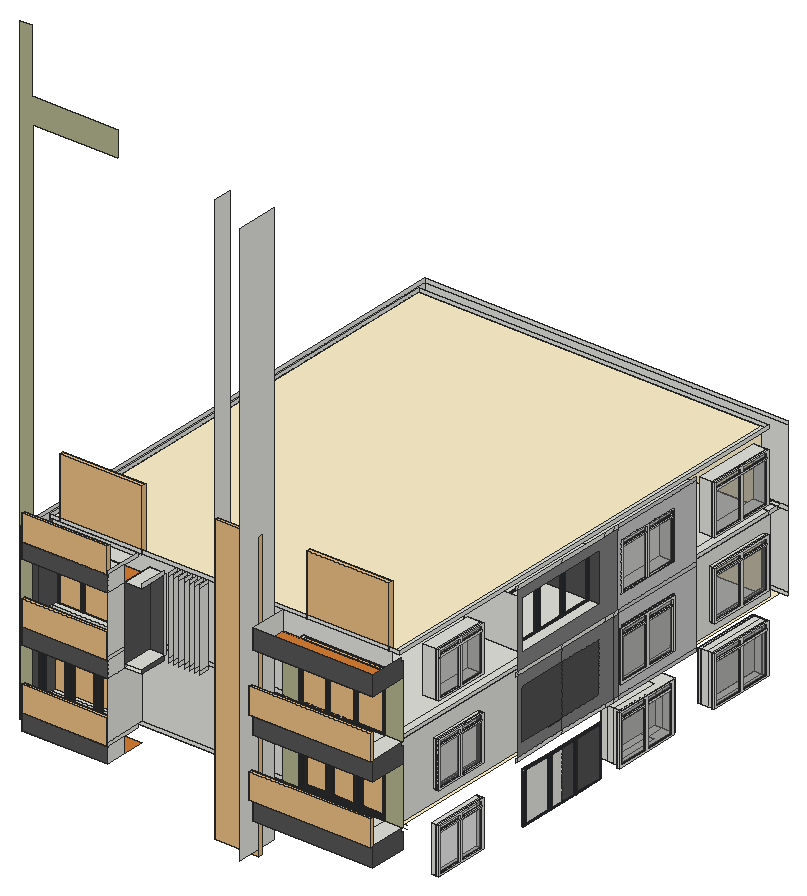
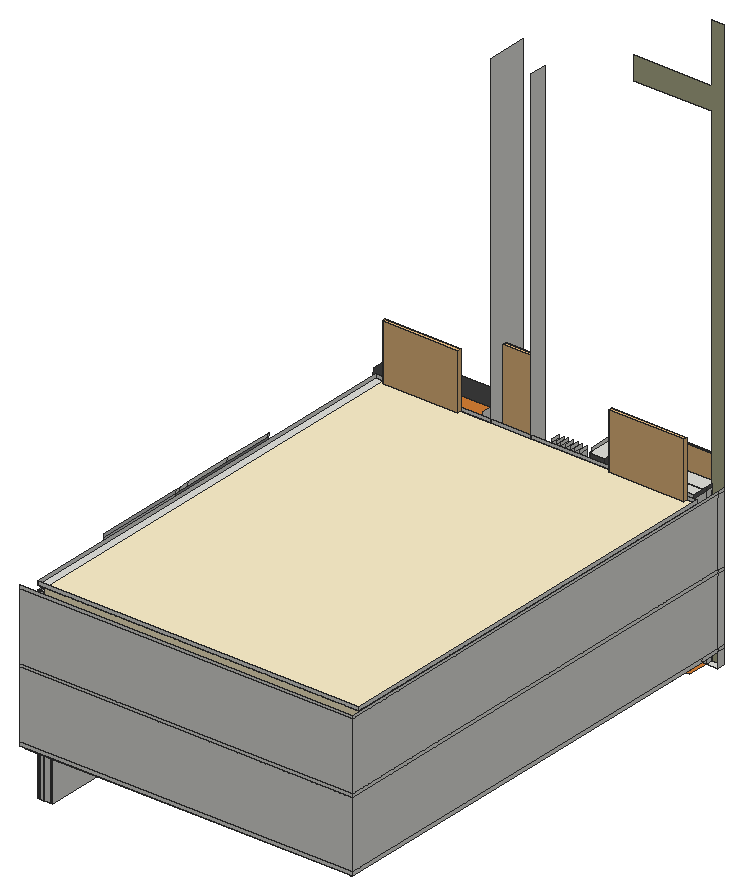
# SketchUp Ruby script. Lengths in inches.
U = 1.inch
M = Sketchup.active_model
def pt(a) = Geom::Point3d.new(a.map { |v| v * U })
def face(e, loops, mat)
  f = e.add_face(loops[0].map { |a| pt(a) })
  loops[1..].each { |l| e.add_face(l.map { |a| pt(a) }).erase! }
  f.material = f.back_material = mat if mat
  f
end
# faces: each face lists its corners as indices into pts; further lists are holes
def faces(e, pts, list, mat = nil) = list.each { |f| face(e, (f[0].is_a?(Array) ? f : [f]).map { |l| l.map { |i| pts[i] } }, mat) }
# xy, xz, yz: faces in a plane at the given z, y or x. An outline is a flat list of corners, or four numbers for a rectangle; further outlines are holes
def ring(l) = l.size == 4 ? [[l[0], l[1]], [l[2], l[1]], [l[2], l[3]], [l[0], l[3]]] : l.each_slice(2).to_a
def flat(e, list, mat, &to3) = list.each { |f| face(e, (f[0].is_a?(Array) ? f : [f]).map { |l| ring(l).map { |u, v| to3.(u, v) } }, mat) }
def xy(e, z, list, mat = nil) = flat(e, list, mat) { |x, y| [x, y, z] }
def xz(e, y, list, mat = nil) = flat(e, list, mat) { |x, z| [x, y, z] }
def yz(e, x, list, mat = nil) = flat(e, list, mat) { |y, z| [x, y, z] }
def lines(e, pts, list) = list.each { |a, b| e.add_line(pt(pts[a]), pt(pts[b])) }
# prism: a flat outline (further loops are holes) pulled along v
def prism(e, loops, v, mat = nil)
  f = face(e, loops, mat); d = Geom::Vector3d.new(v.map { |x| x * U })
  f.pushpull(f.normal.samedirection?(d) ? d.length : -d.length)
end
def box(e, o, s, mat = nil) = prism(e, [[o, [o[0] + s[0], o[1], o[2]], [o[0] + s[0], o[1] + s[1], o[2]], [o[0], o[1] + s[1], o[2]]]], [0, 0, s[2]], mat)
def at(x, y, z, deg = 0) = Geom::Transformation.translation(pt([x, y, z])) * Geom::Transformation.rotation(ORIGIN, Z_AXIS, deg.degrees)
def axes(o, x, y, z) = Geom::Transformation.new([*x, 0, *y, 0, *z, 0, *pt(o).to_a, 1])
def part(name) = M.definitions.add(name)
# library, detail: a bought-in or finely detailed component or shape, given as its bounding box
def library(name, o, s) = part(name).tap { |d| box(d.entities, o, s) }
def detail(e, o, s) = box(e.add_group.entities, o, s)
def put(e, d, t, mat = nil) = e.add_instance(d, t).tap { |i| i.material = mat if mat }
def group(e, t, mat = nil) = e.add_group.tap { |g| g.transformation = t; g.material = mat if mat }.entities
root = M.entities
M.materials.add("Wine2").color = [0, 0, 0]
M.materials["Wine2"].alpha = 0
M.materials.add("[0130_Gainsboro]").color = [39, 45, 50]
M.materials.add("[0133_Gray]").color = [128, 128, 128]
M.materials.add("[0135_DarkGray]1").color = [81, 81, 81]
M.materials.add("[Color D01]").color = [255, 242, 204]
M.materials.add("[Color E01]").color = [178, 178, 142]
M.materials.add("[Color M02]").color = [198, 198, 198]
M.materials.add("[Color M06]").color = [86, 86, 86]
M.materials.add("[Translucent Glass Gray]").color = [128, 128, 128]
M.materials["[Translucent Glass Gray]"].alpha = 0.5
M.materials.add("[Wood Bamboo]").color = [214, 127, 52]
c1 = library("Scandinavian Door w/ Glass Wall\#2",[-41.94,78.85,0],[6.47,62.99,82.68])
c2 = part("Group\#3")
xy(c2.entities,0,[[0,0,32.48,1.97]])
xy(c2.entities,0.98,[[0.98,0,31.5,0.98],[0.98,0.98,31.5,1.97]])
xy(c2.entities,8.86,[[0.98,0,31.5,0.98],[0.98,0.98,31.5,1.97]])
xy(c2.entities,9.84,[[0,0,32.48,1.97]])
xz(c2.entities,0,[[[0,0,32.48,9.84],[0.98,0.98,31.5,8.86]]])
xz(c2.entities,0.98,[[0.98,0.98,31.5,8.86]],"[Translucent Glass Gray]")
xz(c2.entities,1.97,[[[0,0,32.48,9.84],[0.98,0.98,31.5,8.86]]])
yz(c2.entities,0,[[0,0,1.97,9.84]])
yz(c2.entities,0.98,[[0,0.98,0.98,8.86],[0.98,0.98,1.97,8.86]])
yz(c2.entities,31.5,[[0,0.98,0.98,8.86],[0.98,0.98,1.97,8.86]])
yz(c2.entities,32.48,[[0,0,1.97,9.84]])
c3 = part("Group\#4")
xy(c3.entities,0,[[0,0,32.48,1.97]])
xy(c3.entities,0.98,[[0.98,0,31.5,0.98],[0.98,0.98,31.5,1.97]])
xy(c3.entities,71.85,[[0.98,0,31.5,0.98],[0.98,0.98,31.5,1.97]])
xy(c3.entities,72.83,[[0,0,32.48,1.97]])
xz(c3.entities,0,[[[0,0,32.48,72.83],[0.98,0.98,31.5,71.85]]])
xz(c3.entities,0.98,[[0.98,0.98,31.5,71.85]],"[Translucent Glass Gray]")
xz(c3.entities,1.97,[[[0,0,32.48,72.83],[0.98,0.98,31.5,71.85]]])
yz(c3.entities,0,[[0,0,1.97,72.83]])
yz(c3.entities,0.98,[[0,0.98,0.98,71.85],[0.98,0.98,1.97,71.85]])
yz(c3.entities,31.5,[[0,0.98,0.98,71.85],[0.98,0.98,1.97,71.85]])
yz(c3.entities,32.48,[[0,0,1.97,72.83]])
c4 = part("FIXED+GLASS+WINDOW+WITH+TRANSOM")
g1 = group(c4.entities,at(0,0,0))
xy(g1,0,[[0,0,70.86,3.9375]])
xy(g1,1.97,[[1.97,0,34.45,0.98],[36.42,0,68.9,3.9375],[1.97,2.95,34.45,3.9375]])
xy(g1,86.61,[[1.97,0,34.45,3.9375],[34.45,0,36.42,3.9375],[36.42,0,68.9,3.9375]])
xy(g1,88.58,[[0,0,70.86,3.9375]])
xz(g1,0,[[[0,0,70.86,88.58],[1.97,1.97,34.45,86.61],[36.42,1.97,68.9,86.61]]])
xz(g1,3.9375,[[[0,0,70.86,88.58],[1.97,1.97,34.45,86.61],[36.42,1.97,68.9,86.61]]])
yz(g1,0,[[0,0,3.9375,88.58]])
yz(g1,1.97,[[0,1.97,3.9375,74.8],[0,76.77,3.9375,86.61]])
yz(g1,34.45,[[0,1.97,3.9375,86.61]])
yz(g1,36.42,[[0,1.97,3.9375,86.61]])
yz(g1,68.9,[[0,1.97,3.9375,86.61]])
yz(g1,70.86,[[0,0,3.9375,88.58]])
g2 = group(g1,at(1.97,0,74.8))
box(g2,[0,0,0],[66.93,3.9375,1.97])
put(g1,c2,at(1.97,0.98,76.77))
put(g1,c2,at(36.42,0.98,76.77))
put(g1,c3,at(1.97,0.98,1.97))
put(g1,c3,at(36.42,0.98,1.97))
c5 = part("Framed glazing panel")
xy(c5.entities,0,[[0,-0.98,43.07,0],[0,0,43.07,1.4]],"[0130_Gainsboro]")
xy(c5.entities,0.3,[[0.3,-1.43,42.77,-0.98]],"[0130_Gainsboro]")
xy(c5.entities,2.95,[[2.95,-1.43,40.12,-0.63],[2.95,-0.63,40.12,0],[2.95,0,40.12,0.64],[2.95,0.64,40.12,1.4]],"[0130_Gainsboro]")
xy(c5.entities,3.54,[[3.54,-0.63,39.53,0],[3.54,0,39.53,0.64]],"[0130_Gainsboro]")
xy(c5.entities,111.8125,[[3.54,-0.63,39.53,0],[3.54,0,39.53,0.64]],"[0130_Gainsboro]")
xy(c5.entities,112.4,[[2.95,-1.43,40.12,-0.63],[2.95,-0.63,40.12,0],[2.95,0,40.12,0.64],[2.95,0.64,40.12,1.4]],"[0130_Gainsboro]")
xy(c5.entities,115.05,[[0.3,-1.43,42.77,-0.98]],"[0130_Gainsboro]")
xy(c5.entities,115.35,[[0,-0.98,43.07,0],[0,0,43.07,1.4]],"[0130_Gainsboro]")
xz(c5.entities,-1.43,[[[0.3,0.3,42.77,115.05],[2.95,2.95,40.12,112.4]]],"[0130_Gainsboro]")
xz(c5.entities,-0.98,[[[0,0,43.07,115.35],[0.3,0.3,42.77,115.05]]],"[0130_Gainsboro]")
xz(c5.entities,-0.63,[[[2.95,2.95,40.12,112.4],[3.54,3.54,39.53,111.8125]]],"[0130_Gainsboro]")
xz(c5.entities,0,[[3.54,3.54,39.53,111.8125]],"Wine2")
xz(c5.entities,0,[[[0,0,43.07,115.35],[2.95,2.95,40.12,112.4]],[[2.95,2.95,40.12,112.4],[3.54,3.54,39.53,111.8125]]],"[0130_Gainsboro]")
xz(c5.entities,0.64,[[[2.95,2.95,40.12,112.4],[3.54,3.54,39.53,111.8125]]],"[0130_Gainsboro]")
xz(c5.entities,1.4,[[[0,0,43.07,115.35],[2.95,2.95,40.12,112.4]]],"[0130_Gainsboro]")
yz(c5.entities,0,[[-0.98,0,0,115.35],[0,0,1.4,115.35]],"[0130_Gainsboro]")
yz(c5.entities,0.3,[[-1.43,0.3,-0.98,115.05]],"[0130_Gainsboro]")
yz(c5.entities,2.95,[[-1.43,2.95,-0.63,112.4],[-0.63,2.95,0,112.4],[0,2.95,0.64,112.4],[0.64,2.95,1.4,112.4]],"[0130_Gainsboro]")
yz(c5.entities,3.54,[[-0.63,3.54,0,111.8125],[0,3.54,0.64,111.8125]],"[0130_Gainsboro]")
yz(c5.entities,39.53,[[-0.63,3.54,0,111.8125],[0,3.54,0.64,111.8125]],"[0130_Gainsboro]")
yz(c5.entities,40.12,[[-1.43,2.95,-0.63,112.4],[-0.63,2.95,0,112.4],[0,2.95,0.64,112.4],[0.64,2.95,1.4,112.4]],"[0130_Gainsboro]")
yz(c5.entities,42.77,[[-1.43,0.3,-0.98,115.05]],"[0130_Gainsboro]")
yz(c5.entities,43.07,[[-0.98,0,0,115.35],[0,0,1.4,115.35]],"[0130_Gainsboro]")
c6 = part("Glazing assembly")
put(c6.entities,c5,axes([90.57,1.43,0],[1.05148,0,0],[0,1,0],[0,0,1]))
put(c6.entities,c5,axes([0,1.43,0],[1.05148,0,0],[0,1,0],[0,0,1]))
put(c6.entities,c5,axes([45.29,1.43,0],[1.05148,0,0],[0,1,0],[0,0,1]))
c7 = library("Group5_1",[-7.56,-66.38,0.11],[6.33,135.04,120.95])
c8 = library("Glass Railing",[0,0,0],[139.5,4.76,42])
xy(root,270.83,[[706.43,942.08,709.93,1053.14],[709.93,942.08,721.74,1052.58],[721.74,942.08,733.4375,1053.14],[709.93,1052.58,721.74,1053.14]])
xy(root,271.38,[[700.49,750.25,711.3,832.49],[711.3,750.25,721.74,832.49],[721.74,750.25,733.4375,750.25,733.4375,861.32,711.3,861.32,711.3,832.49,721.74,832.49],[700.49,832.49,711.3,861.32]])
xy(root,274.03,[[721.74,375.23,733.4375,467.6]])
xy(root,279.6,[[442.42,279.375,514.85,310.82]])
xy(root,345.6875,[[137.375,261.5,157.82,273.3125],[563.32,301.625,704.2,310.82]])
xy(root,345.6875,[[157.82,240.3125,298.7,273.3125],[536.21,240.3125,733.4375,301.625],[157.82,273.3125,298.7,310.82]],"[Wood Bamboo]")
xy(root,348.53,[[721.74,375.23,733.4375,467.6]])
xy(root,352.08,[[706.43,942.08,709.93,1053.14],[709.93,942.08,721.74,1052.58],[721.74,942.08,733.4375,1053.14],[709.93,1052.58,721.74,1053.14]])
xy(root,352.63,[[700.49,750.25,711.3,832.49],[711.3,750.25,721.74,832.49],[721.74,750.25,721.74,832.49,711.3,832.49,711.3,861.32,733.4375,861.32,733.4375,750.25],[700.49,832.49,711.3,861.32]])
xy(root,371.625,[[157.82,240.3125,298.7,273.3125],[157.82,273.3125,298.7,301.625],[137.375,1091.875,721.74,1092.875]])
xy(root,371.625,[[137.375,310.82,721.74,1091.875]],"[Color D01]")
xy(root,377.625,[[536.21,240.3125,563.32,301.625],[563.32,240.3125,704.2,310.82],[704.2,240.3125,733.4375,301.625],[157.82,301.625,298.7,310.82],[146.57,310.82,721.74,1067.8],
  [721.74,310.82,723.55,1067.8]])
xy(root,396.83,[[721.74,942.08,723.55,1053.14],[723.55,942.08,733.4375,1053.14]])
xy(root,397.38,[[728.75,750.25,733.4375,861.32]])
xy(root,400.03,[[721.74,375.23,723.55,467.6],[723.55,375.23,733.4375,467.6]])
xy(root,471.6875,[[563.32,301.625,704.2,310.82]])
xy(root,471.6875,[[157.82,240.3125,298.7,273.3125],[536.21,240.3125,733.4375,301.625],[157.82,273.3125,298.7,310.82]],"[Wood Bamboo]")
xy(root,474.53,[[721.74,375.23,723.55,467.6],[723.55,375.23,733.4375,467.6]])
xy(root,478.08,[[721.74,942.08,723.55,1053.14],[723.55,942.08,733.4375,1053.14]])
xy(root,478.63,[[728.75,750.25,733.4375,861.32]])
xy(root,497.625,[[326.68,240.0625,354.04,279.375],[157.82,240.3125,298.7,273.3125],[157.82,273.3125,298.7,301.625],[721.74,310.82,723.55,1067.8],[146.57,1067.8,721.74,1083.67],
  [146.57,1083.67,721.74,1091.875]])
xy(root,497.625,[[146.57,310.82,721.74,1067.8]],"[Color D01]")
xy(root,503.625,[[326.68,240.0625,354.04,290.5],[536.21,240.3125,563.32,301.625],[563.32,240.3125,704.2,310.82],[704.2,240.3125,733.4375,301.625],[157.82,301.625,298.7,310.82],
  [146.57,310.82,708.49,1067.8],[708.49,310.82,721.74,1067.8],[146.57,1067.8,708.49,1083.67],[708.49,1067.8,721.74,1083.67],[146.57,1083.67,708.49,1091.875],
  [708.49,1083.67,721.74,1091.875]])
xy(root,522.83,[[708.49,942.08,733.4375,1053.14]])
xy(root,523.38,[[708.49,750.25,733.4375,861.32]])
xy(root,528.26,[[639.1875,545.74,733.4375,707.42]])
xy(root,532.03,[[708.49,375.23,733.4375,467.6]])
xy(root,597.6875,[[563.32,301.625,704.2,310.82]])
xy(root,597.6875,[[157.82,240.3125,298.7,273.3125],[536.21,240.3125,733.4375,301.625],[157.82,273.3125,298.7,310.82]],"[Wood Bamboo]")
xy(root,604.08,[[708.49,942.08,733.4375,1053.14]])
xy(root,604.63,[[708.49,750.25,733.4375,861.32]])
xy(root,606.53,[[708.49,375.23,733.4375,467.6]])
xy(root,608.63,[[639.1875,545.74,733.4375,707.42]])
xy(root,623.625,[[326.68,240.0625,354.04,290.5],[157.82,240.3125,298.7,273.3125],[157.82,273.3125,298.7,301.625],[708.49,310.82,721.74,1067.8]])
xy(root,623.625,[[146.57,310.82,708.49,1067.8]],"[Color D01]")
xz(root,240.3125,[[157.82,345.6875,298.7,371.625],[536.21,345.6875,733.4375,377.625],[157.82,471.6875,298.7,497.625],[536.21,471.6875,733.4375,503.625],[157.82,597.6875,298.7,623.625],
  [536.21,597.6875,733.4375,629.625]],"[Color M06]")
xz(root,261.5,[[137.375,345.6875,157.82,345.6875,157.82,1227.6875,298.7,1227.6875,298.7,1269.0625,157.51,1269.0625,157.51,1373.625,137.375,1373.625]],"[Color E01]")
xz(root,273.3125,[[157.82,345.6875,298.7,371.625],[157.82,471.6875,298.7,497.625],[157.82,597.6875,298.7,623.625]])
xz(root,290.5,[[326.68,503.625,354.04,623.625]],"[Color M06]")
xz(root,301.625,[[157.82,371.625,298.7,377.625],[157.82,497.625,298.7,503.625],[157.82,623.625,298.7,629.625]])
xz(root,301.625,[[536.21,377.625,563.32,471.6875],[704.2,377.625,733.4375,471.6875],[536.21,503.625,563.32,597.6875],[704.2,503.625,733.4375,597.6875]],"[Color E01]")
xz(root,310.82,[[137.375,371.625,146.57,377.625],[146.57,371.625,442.42,377.625],[442.42,371.625,514.85,377.625],[514.85,371.625,721.74,377.625],[146.57,377.625,146.57,497.625,442.42,497.625,442.42,377.625,298.7,377.625,298.7,471.6875,157.82,471.6875,157.82,377.625],
  [514.85,377.625,514.85,497.625,721.74,497.625,721.74,377.625,704.2,377.625,704.2,471.6875,563.32,471.6875,563.32,377.625],[721.74,377.625,723.55,497.625],[146.57,497.625,442.42,503.625],[442.42,497.625,514.85,503.625],[514.85,497.625,721.74,503.625],
  [146.57,503.625,146.57,623.625,442.42,623.625,442.42,503.625,298.7,503.625,298.7,597.6875,157.82,597.6875,157.82,503.625],[514.85,503.625,514.85,623.625,708.49,623.625,708.49,503.625,704.2,503.625,704.2,597.6875,563.32,597.6875,563.32,503.625],[146.57,623.625,442.42,629.625],[442.42,623.625,514.85,629.625],[514.85,623.625,721.74,629.625]])
xz(root,375.23,[[721.74,274.03,733.4375,348.53],[721.74,400.03,723.55,474.53],[723.55,400.03,733.4375,474.53],[708.49,532.03,733.4375,606.53]])
xz(root,467.6,[[721.74,274.03,733.4375,348.53],[721.74,400.03,723.55,474.53],[723.55,400.03,733.4375,474.53],[708.49,532.03,733.4375,606.53]])
xz(root,545.74,[[639.1875,528.26,733.4375,608.63]])
xz(root,707.42,[[639.1875,528.26,733.4375,608.63]],"[0135_DarkGray]1")
xz(root,750.25,[[700.49,271.38,711.3,352.63],[711.3,271.38,721.74,352.63],[721.74,271.38,733.4375,352.63],[728.75,397.38,733.4375,478.63],[708.49,523.38,733.4375,604.63]])
xz(root,861.32,[[700.49,271.38,711.3,352.63],[711.3,271.38,733.4375,352.63],[728.75,397.38,733.4375,478.63],[708.49,523.38,733.4375,604.63]])
xz(root,942.08,[[706.43,270.83,709.93,352.08],[709.93,270.83,721.74,352.08],[721.74,270.83,733.4375,352.08],[721.74,396.83,723.55,478.08],[723.55,396.83,733.4375,478.08],
  [708.49,522.83,733.4375,604.08]])
xz(root,1052.58,[[709.93,270.83,721.74,352.08]])
xz(root,1053.14,[[706.43,270.83,709.93,352.08],[709.93,270.83,721.74,352.08],[721.74,270.83,733.4375,352.08],[721.74,396.83,723.55,478.08],[723.55,396.83,733.4375,478.08],
  [708.49,522.83,733.4375,604.08]])
xz(root,1067.8,[[721.74,377.625,723.55,497.625],[146.57,497.625,721.74,503.625],[146.57,623.625,721.74,629.625]])
xz(root,1067.8,[[146.57,377.625,721.74,497.625],[146.57,503.625,708.49,623.625]],"[Color D01]")
xz(root,1083.67,[[146.57,497.625,721.74,503.625]])
xz(root,1091.875,[[137.375,371.625,733.4375,377.625],[137.375,377.625,733.4375,497.625],[137.375,497.625,733.4375,503.625],[137.375,503.625,733.4375,623.625],[137.375,623.625,733.4375,629.625]])
yz(root,137.375,[[261.5,345.6875,273.3125,371.625],[261.5,371.625,273.3125,377.625],[273.3125,371.625,310.82,377.625],[310.82,371.625,1091.875,377.625],[261.5,377.625,273.3125,497.625],
  [273.3125,377.625,1091.875,497.625],[261.5,497.625,273.3125,503.625],[273.3125,497.625,1091.875,503.625],[261.5,503.625,273.3125,623.625],[273.3125,503.625,1091.875,623.625],
  [261.5,623.625,273.3125,629.625],[273.3125,623.625,1091.875,629.625]])
yz(root,146.57,[[310.82,497.625,1067.8,503.625],[1067.8,497.625,1083.67,503.625],[310.82,623.625,1067.8,629.625]])
yz(root,146.57,[[310.82,377.625,1067.8,497.625],[310.82,503.625,1067.8,623.625]],"[Color D01]")
yz(root,157.82,[[240.3125,345.6875,261.5,371.625],[261.5,345.6875,273.3125,371.625],[261.5,371.625,273.3125,377.625],[273.3125,371.625,301.625,377.625],[240.3125,471.6875,261.5,497.625],
  [261.5,471.6875,273.3125,497.625],[261.5,497.625,273.3125,503.625],[273.3125,497.625,301.625,503.625],[240.3125,597.6875,261.5,623.625],[261.5,597.6875,273.3125,623.625]])
yz(root,157.82,[[261.5,377.625,273.3125,471.6875],[273.3125,377.625,310.82,471.6875],[261.5,503.625,273.3125,597.6875],[273.3125,503.625,310.82,597.6875],[261.5,623.625,273.3125,629.625],
  [273.3125,623.625,301.625,629.625]],"[Color M06]")
yz(root,298.7,[[240.0625,345.6875,240.3125,371.625],[240.3125,345.6875,273.3125,371.625],[240.0625,371.625,301.625,377.625],[240.0625,377.625,310.82,471.6875],[240.0625,471.6875,240.3125,497.625],
  [240.3125,471.6875,273.3125,497.625],[240.0625,497.625,301.625,503.625],[240.0625,503.625,310.82,597.6875],[240.0625,597.6875,240.3125,623.625],[240.3125,597.6875,273.3125,623.625],
  [240.0625,623.625,301.625,629.625]])
yz(root,326.68,[[240.0625,503.625,290.5,623.625]],"[Color M06]")
yz(root,354.04,[[285.875,503.625,290.5,623.625],[240.0625,623.625,285.875,629.625]])
yz(root,354.04,[[240.0625,497.625,285.875,503.625]],"[Color M06]")
yz(root,362.47,[[285.875,497.625,301.625,503.625],[285.875,503.625,301.625,623.625],[285.875,623.625,301.625,629.625]])
yz(root,370.91,[[285.875,497.625,301.625,503.625],[285.875,503.625,301.625,623.625],[285.875,623.625,301.625,629.625]])
yz(root,379.35,[[285.875,497.625,301.625,503.625],[285.875,503.625,301.625,623.625],[285.875,623.625,301.625,629.625]])
yz(root,387.79,[[285.875,497.625,301.625,503.625],[285.875,503.625,301.625,623.625],[285.875,623.625,301.625,629.625]])
yz(root,396.22,[[285.875,497.625,301.625,503.625],[285.875,503.625,301.625,623.625],[285.875,623.625,301.625,629.625]])
yz(root,404.66,[[285.875,497.625,301.625,503.625],[285.875,503.625,301.625,623.625],[285.875,623.625,301.625,629.625]])
yz(root,413.1,[[285.875,497.625,301.625,503.625],[285.875,503.625,301.625,623.625],[285.875,623.625,301.625,629.625]])
yz(root,442.42,[[279.375,279.6,310.82,1208.73]])
yz(root,514.85,[[240.0625,279.6,310.82,1208.73]])
yz(root,536.21,[[240.3125,345.6875,301.625,377.625],[240.3125,471.6875,301.625,503.625],[240.3125,597.6875,301.625,629.625]])
yz(root,563.32,[[301.625,377.625,310.82,471.6875],[301.625,503.625,310.82,597.6875]])
yz(root,639.1875,[[545.74,528.26,707.42,608.63]],"[0135_DarkGray]1")
yz(root,700.49,[[750.25,271.38,861.32,352.63]])
yz(root,704.2,[[301.625,377.625,310.82,471.6875],[301.625,503.625,310.82,597.6875]])
yz(root,706.43,[[942.08,270.83,1053.14,352.08]])
yz(root,709.93,[[942.08,270.83,1052.58,352.08],[1052.58,270.83,1053.14,352.08]])
yz(root,721.74,[[1052.58,270.83,1053.14,352.08],[[310.82,377.625,1067.8,497.625],[942.08,396.83,1053.14,478.08],[375.23,400.03,467.6,474.53]],[310.82,497.625,1067.8,503.625],[1067.8,497.625,1083.67,503.625],[310.82,623.625,1067.8,629.625]])
yz(root,723.55,[[[310.82,377.625,1067.8,497.625],[942.08,396.83,1053.14,478.08],[375.23,400.03,467.6,474.53]]])
yz(root,733.4375,[[549.1,270.75,628.83,353.62],[534.42,371.625,537.75,377.625],[537.75,371.625,628.83,377.625],[628.83,371.625,716.73,377.625],[716.73,371.625,735.26,377.625],
  [735.26,371.625,744.22,377.625],[534.42,497.625,537.75,503.625],[537.75,497.625,628.83,503.625],[628.83,497.625,716.73,503.625],[716.73,497.625,735.26,503.625],
  [735.26,497.625,744.22,503.625],[534.42,623.625,537.75,629.625],[537.75,623.625,628.83,629.625],[628.83,623.625,716.73,629.625],[716.73,623.625,735.26,629.625],
  [735.26,623.625,744.22,629.625]])
yz(root,733.4375,[[537.75,377.625,628.83,377.625,628.83,396.33,546.82,396.33,546.82,478.02,628.83,478.02,628.83,497.625,537.75,497.625],[628.83,377.625,735.26,377.625,735.26,497.625,628.83,497.625,628.83,478.02,704.2,478.02,704.2,396.33,628.83,396.33],[735.26,377.625,744.22,497.625],[[537.75,503.625,744.22,623.625],[545.74,528.26,707.42,608.63]]],"[0133_Gray]")
yz(root,733.4375,[[628.83,270.75,709.1,353.62],[546.82,396.33,628.83,478.02],[628.83,396.33,704.2,478.02]],"[0135_DarkGray]1")
yz(root,733.4375,[[744.22,371.625,904.3,377.625],[[744.22,377.625,904.3,497.625],[750.25,397.38,861.32,478.63]],[744.22,497.625,904.3,503.625],[[744.22,503.625,904.3,623.625],[750.25,523.38,861.32,604.63]],[744.22,623.625,904.3,629.625]],"[Color M02]")
yz(root,733.4375,[[549.1,270.75,628.83,353.62],[240.3125,345.6875,301.625,345.6875,301.625,371.625,297.25,371.625,297.25,377.625,240.3125,377.625],[240.3125,471.6875,301.625,471.6875,301.625,497.625,298.875,497.625,298.875,503.625,240.3125,503.625],[240.3125,597.6875,301.625,597.6875,301.625,623.625,298.875,623.625,298.875,629.625,240.3125,629.625]],"[Color M06]")
p = [[728.75,750.25,397.38],[712.375,750.25,397.38],[728.75,861.32,397.38],[712.375,861.32,397.38],[728.75,861.32,478.63],[712.375,861.32,478.63],
  [733.4375,310.82,371.625],[721.74,310.82,371.625],[733.4375,310.82,377.625],[723.55,310.82,377.625]]
lines(root,p,[[0,1],[2,3],[4,5],[6,7],[8,9]])
put(root,c1,axes([350.96,243.91,268.61],[0,-1,0],[1.16,0,0],[0,0,5.69]))
put(root,c4,axes([733.4375,747.17,269.58],[0,1.56726,0],[-1,0,0],[0,0,0.91722]))
put(root,c6,axes([733.81,550.06,270.75],[0,1.17066,0],[-1.13,0,0],[0,0,0.72061]))
put(root,c4,axes([733.4375,942.08,270.83],[0,1.56726,0],[-1,0,0],[0,0,0.91722]))
put(root,c4,axes([733.4375,375.23,274.03],[0,1.30355,0],[-1,0,0],[0,0,0.84102]))
put(root,c7,axes([222.85,306.6875,371.02],[0,-1,0],[1,0,0],[0,0,0.83156]))
put(root,c7,axes([635.54,309.6,371.02],[0,-1,0],[1,0,0],[0,0,0.83156]))
put(root,c8,at(157.82,240.3125,371.625))
put(root,c6,axes([157.82,285.125,371.625],[1.03691,0,0],[0,-4,0],[0,0,0.80657]),"[Color M06]")
put(root,c6,axes([563.32,312.95,377.625],[1.03691,0,0],[0,-4,0],[0,0,0.80657]))
put(root,c8,axes([534.23,235.55,377.625],[1.428,0,0],[0,1,0],[0,0,1]))
put(root,c6,axes([733.4375,548.78,394.2],[0,1.17066,0],[-1.13,0,0],[0,0,0.72061]))
put(root,c4,axes([736.39,745.63,394.68],[0,1.56726,0],[-1,0,0],[0,0,0.91722]))
put(root,c4,axes([733.4375,942.08,396.83],[0,1.56726,0],[-1,0,0],[0,0,0.91722]))
put(root,c4,axes([733.4375,375.23,400.03],[0,1.30355,0],[-1,0,0],[0,0,0.84102]))
put(root,c7,axes([635.54,300.4,497.02],[0,-1,0],[1,0,0],[0,0,0.83156]))
put(root,c7,axes([230.04,309.6,497.02],[0,-1,0],[1,0,0],[0,0,0.83156]))
put(root,c8,at(157.82,240.3125,497.625))
put(root,c6,axes([154.6,322.15,501.24],[1.03691,0,0],[0,-4,0],[0,0,0.80657]))
put(root,c6,axes([563.32,312.95,503.625],[1.03691,0,0],[0,-4,0],[0,0,0.80657]))
put(root,c8,axes([534.23,235.55,503.625],[1.428,0,0],[0,1,0],[0,0,1]))
put(root,c4,axes([733.4375,942.08,522.83],[0,1.56726,0],[-1,0,0],[0,0,0.91722]))
put(root,c4,axes([733.4375,750.25,523.38],[0,1.56726,0],[-1,0,0],[0,0,0.91722]))
put(root,c6,axes([715.0625,548.78,526.13],[0,1.17066,0],[-1.13,0,0],[0,0,0.72061]))
put(root,c4,axes([733.4375,375.23,532.03],[0,1.30355,0],[-1,0,0],[0,0,0.84102]))
put(root,c7,axes([230.04,309.6,623.02],[0,-1,0],[1,0,0],[0,0,0.83156]))
put(root,c7,axes([635.54,309.6,623.02],[0,-1,0],[1,0,0],[0,0,0.83156]))
put(root,c8,at(157.82,240.3125,623.625))
